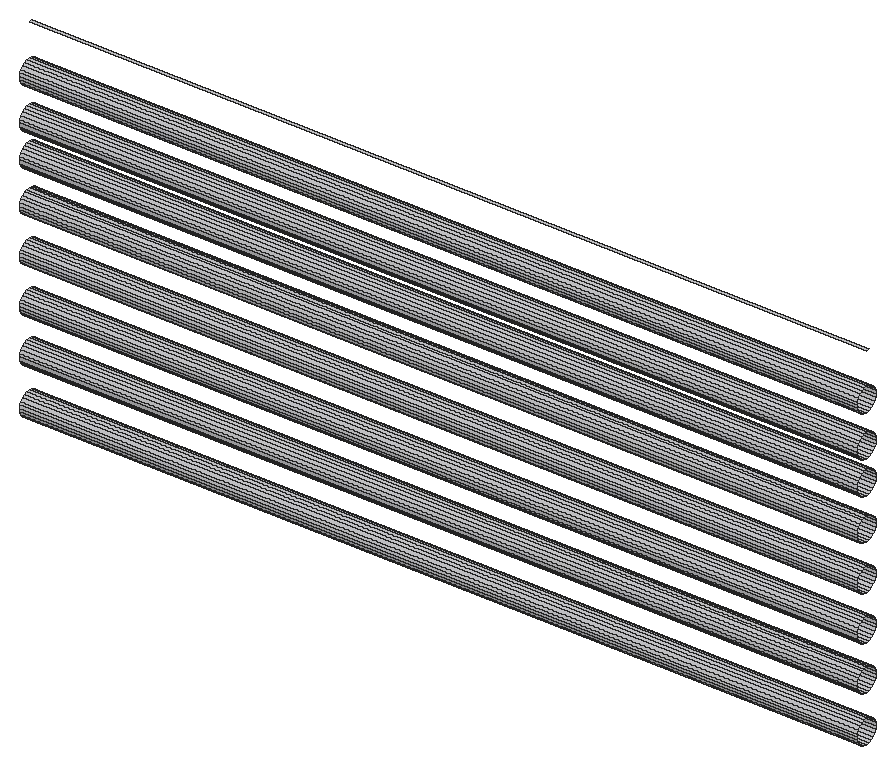
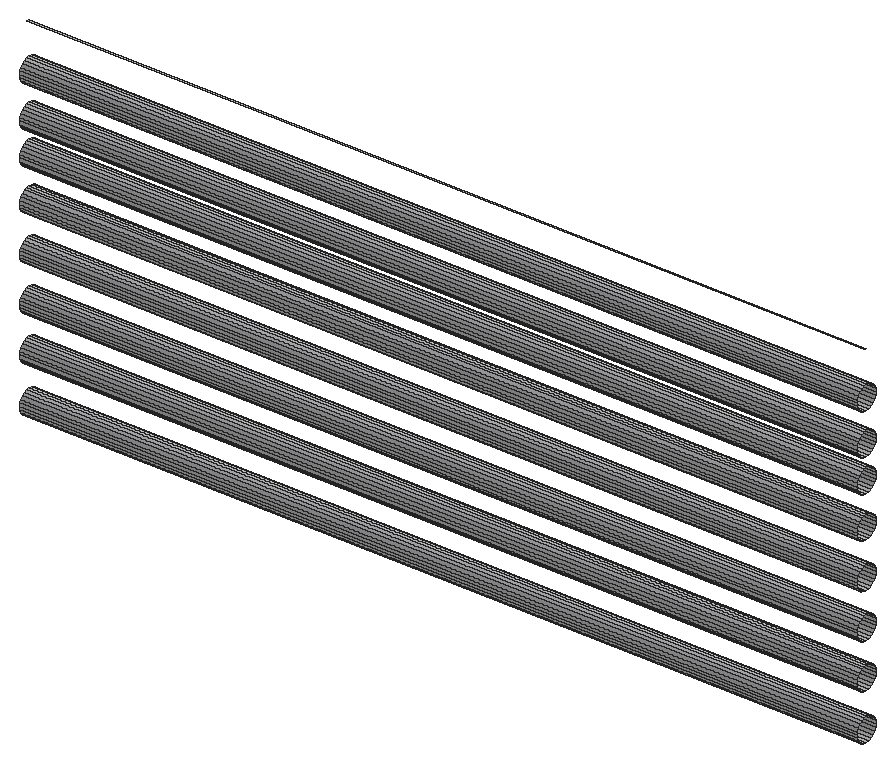
# SketchUp Ruby script. Lengths in inches.
U = 1.inch
M = Sketchup.active_model
def pt(a) = Geom::Point3d.new(a.map { |v| v * U })
def face(e, loops, mat)
  f = e.add_face(loops[0].map { |a| pt(a) })
  loops[1..].each { |l| e.add_face(l.map { |a| pt(a) }).erase! }
  f.material = f.back_material = mat if mat
  f
end
# faces: each face lists its corners as indices into pts; further lists are holes
def faces(e, pts, list, mat = nil) = list.each { |f| face(e, (f[0].is_a?(Array) ? f : [f]).map { |l| l.map { |i| pts[i] } }, mat) }
# xy, xz, yz: faces in a plane at the given z, y or x. An outline is a flat list of corners, or four numbers for a rectangle; further outlines are holes
def ring(l) = l.size == 4 ? [[l[0], l[1]], [l[2], l[1]], [l[2], l[3]], [l[0], l[3]]] : l.each_slice(2).to_a
def flat(e, list, mat, &to3) = list.each { |f| face(e, (f[0].is_a?(Array) ? f : [f]).map { |l| ring(l).map { |u, v| to3.(u, v) } }, mat) }
def xy(e, z, list, mat = nil) = flat(e, list, mat) { |x, y| [x, y, z] }
def xz(e, y, list, mat = nil) = flat(e, list, mat) { |x, z| [x, y, z] }
def yz(e, x, list, mat = nil) = flat(e, list, mat) { |y, z| [x, y, z] }
def lines(e, pts, list) = list.each { |a, b| e.add_line(pt(pts[a]), pt(pts[b])) }
# prism: a flat outline (further loops are holes) pulled along v
def prism(e, loops, v, mat = nil)
  f = face(e, loops, mat); d = Geom::Vector3d.new(v.map { |x| x * U })
  f.pushpull(f.normal.samedirection?(d) ? d.length : -d.length)
end
def box(e, o, s, mat = nil) = prism(e, [[o, [o[0] + s[0], o[1], o[2]], [o[0] + s[0], o[1] + s[1], o[2]], [o[0], o[1] + s[1], o[2]]]], [0, 0, s[2]], mat)
def at(x, y, z, deg = 0) = Geom::Transformation.translation(pt([x, y, z])) * Geom::Transformation.rotation(ORIGIN, Z_AXIS, deg.degrees)
def axes(o, x, y, z) = Geom::Transformation.new([*x, 0, *y, 0, *z, 0, *pt(o).to_a, 1])
def part(name) = M.definitions.add(name)
# library, detail: a bought-in or finely detailed component or shape, given as its bounding box
def library(name, o, s) = part(name).tap { |d| box(d.entities, o, s) }
def detail(e, o, s) = box(e.add_group.entities, o, s)
def put(e, d, t, mat = nil) = e.add_instance(d, t).tap { |i| i.material = mat if mat }
def group(e, t, mat = nil) = e.add_group.tap { |g| g.transformation = t; g.material = mat if mat }.entities
root = M.entities
M.materials.add("[Polished Concrete New]").color = [200, 200, 203]
p = [[204.4,120.13,10.75],[204.4,119.98,10.8125],[160.24,119.98,10.8125],[160.24,120.13,10.75],[204.4,120.29,10.73],[160.24,120.29,10.73],
  [204.4,120.45,10.75],[160.24,120.45,10.75],[204.4,120.6,10.8125],[160.24,120.6,10.8125],[204.4,119.85,10.91],[160.24,119.85,10.91],
  [204.4,120.73,10.91],[160.24,120.73,10.91],[204.4,119.75,11.04],[160.24,119.75,11.04],[204.4,120.83,11.04],[160.24,120.83,11.04],
  [204.4,119.6875,11.19],[160.24,119.6875,11.19],[204.4,120.89,11.19],[160.24,120.89,11.19],[204.4,119.66,11.35],[160.24,119.66,11.35],
  [204.4,120.91,11.35],[160.24,120.91,11.35],[204.4,119.6875,11.51],[160.24,119.6875,11.51],[204.4,120.89,11.51],[160.24,120.89,11.51],
  [204.4,119.75,11.66],[160.24,119.75,11.66],[204.4,120.83,11.66],[160.24,120.83,11.66],[204.4,119.85,11.79],[160.24,119.85,11.79],
  [204.4,120.73,11.79],[160.24,120.73,11.79],[204.4,119.98,11.89],[160.24,119.98,11.89],[204.4,120.6,11.89],[160.24,120.6,11.89],
  [204.4,120.13,11.96],[160.24,120.13,11.96],[204.4,120.45,11.96],[160.24,120.45,11.96],[204.4,120.29,11.98],[160.24,120.29,11.98],
  [204.4,119.98,13.25],[204.4,119.85,13.35],[160.24,119.85,13.35],[160.24,119.98,13.25],[204.4,120.13,13.1875],[160.24,120.13,13.1875],
  [204.4,120.29,13.16],[160.24,120.29,13.16],[204.4,120.45,13.1875],[160.24,120.45,13.1875],[204.4,120.6,13.25],[160.24,120.6,13.25],
  [204.4,120.73,13.35],[160.24,120.73,13.35],[204.4,119.75,13.48],[160.24,119.75,13.48],[204.4,120.83,13.48],[160.24,120.83,13.48],
  [204.4,119.6875,13.63],[160.24,119.6875,13.63],[204.4,120.89,13.63],[160.24,120.89,13.63],[204.4,119.66,13.79],[160.24,119.66,13.79],
  [204.4,120.91,13.79],[160.24,120.91,13.79],[204.4,119.6875,13.95],[160.24,119.6875,13.95],[204.4,120.89,13.95],[160.24,120.89,13.95],
  [204.4,119.75,14.1],[160.24,119.75,14.1],[204.4,120.83,14.1],[160.24,120.83,14.1],[204.4,119.85,14.23],[160.24,119.85,14.23],
  [204.4,120.73,14.23],[160.24,120.73,14.23],[204.4,119.98,14.33],[160.24,119.98,14.33],[204.4,120.6,14.33],[160.24,120.6,14.33],
  [204.4,120.13,14.39],[160.24,120.13,14.39],[204.4,120.45,14.39],[160.24,120.45,14.39],[204.4,120.29,14.41],[160.24,120.29,14.41],
  [204.4,120.29,15.54],[204.4,120.13,15.5625],[160.24,120.13,15.5625],[160.24,120.29,15.54],[204.4,120.45,15.5625],[160.24,120.45,15.5625],
  [204.4,119.98,15.625],[204.4,119.85,15.72],[160.24,119.85,15.72],[160.24,119.98,15.625],[204.4,120.6,15.625],[160.24,120.6,15.625],
  [204.4,120.73,15.72],[160.24,120.73,15.72],[204.4,119.75,15.85],[160.24,119.75,15.85],[204.4,120.83,15.85],[160.24,120.83,15.85],
  [204.4,119.6875,16],[160.24,119.6875,16],[204.4,120.89,16],[160.24,120.89,16],[204.4,119.66,16.16],[160.24,119.66,16.16],
  [204.4,120.91,16.16],[160.24,120.91,16.16],[204.4,119.6875,16.33],[160.24,119.6875,16.33],[204.4,120.89,16.33],[160.24,120.89,16.33],
  [204.4,119.75,16.48],[160.24,119.75,16.48],[204.4,120.83,16.48],[160.24,120.83,16.48],[204.4,119.85,16.61],[160.24,119.85,16.61],
  [204.4,120.73,16.61],[160.24,120.73,16.61],[204.4,119.98,16.71],[160.24,119.98,16.71],[204.4,120.6,16.71],[160.24,120.6,16.71],
  [204.4,120.13,16.77],[160.24,120.13,16.77],[204.4,120.45,16.77],[160.24,120.45,16.77],[204.4,120.29,16.79],[160.24,120.29,16.79],
  [204.4,120.13,17.9375],[204.4,119.98,18],[160.24,119.98,18],[160.24,120.13,17.9375],[204.4,120.29,17.91],[160.24,120.29,17.91],
  [204.4,120.45,17.9375],[160.24,120.45,17.9375],[204.4,120.6,18],[160.24,120.6,18],[204.4,119.85,18.1],[160.24,119.85,18.1],
  [204.4,120.73,18.1],[160.24,120.73,18.1],[204.4,119.75,18.23],[160.24,119.75,18.23],[204.4,120.83,18.23],[160.24,120.83,18.23],
  [204.4,119.6875,18.38],[160.24,119.6875,18.38],[204.4,120.89,18.38],[160.24,120.89,18.38],[204.4,119.66,18.54],[160.24,119.66,18.54],
  [204.4,120.91,18.54],[160.24,120.91,18.54],[204.4,119.6875,18.7],[160.24,119.6875,18.7],[204.4,120.89,18.7],[160.24,120.89,18.7],
  [204.4,119.75,18.85],[160.24,119.75,18.85],[204.4,120.83,18.85],[160.24,120.83,18.85],[204.4,119.85,18.98],[160.24,119.85,18.98],
  [204.4,120.73,18.98],[160.24,120.73,18.98],[204.4,119.98,19.08],[160.24,119.98,19.08],[204.4,120.6,19.08],[160.24,120.6,19.08],
  [204.4,120.13,19.14],[160.24,120.13,19.14],[204.4,120.29,19.16],[160.24,120.29,19.16],[204.4,120.45,19.14],[160.24,120.45,19.14],
  [204.4,120.13,20.3125],[204.4,119.98,20.375],[160.24,119.98,20.375],[160.24,120.13,20.3125],[204.4,120.29,20.29],[160.24,120.29,20.29],
  [204.4,120.45,20.3125],[160.24,120.45,20.3125],[204.4,120.6,20.375],[160.24,120.6,20.375],[204.4,119.85,20.47],[160.24,119.85,20.47],
  [204.4,120.73,20.47],[160.24,120.73,20.47],[204.4,119.75,20.6],[160.24,119.75,20.6],[204.4,120.83,20.6],[160.24,120.83,20.6],
  [204.4,119.6875,20.75],[160.24,119.6875,20.75],[204.4,120.89,20.75],[160.24,120.89,20.75],[204.4,119.66,20.91],[160.24,119.66,20.91],
  [204.4,120.91,20.91],[160.24,120.91,20.91],[204.4,119.6875,21.08],[160.24,119.6875,21.08],[204.4,120.89,21.08],[160.24,120.89,21.08],
  [204.4,119.75,21.23],[160.24,119.75,21.23],[204.4,120.83,21.23],[160.24,120.83,21.23],[204.4,119.85,21.36],[160.24,119.85,21.36],
  [204.4,120.73,21.36],[160.24,120.73,21.36],[204.4,119.98,21.46],[160.24,119.98,21.46],[204.4,120.6,21.46],[160.24,120.6,21.46],
  [204.4,120.13,21.52],[160.24,120.13,21.52],[204.4,120.29,21.54],[160.24,120.29,21.54],[204.4,120.45,21.52],[160.24,120.45,21.52],
  [204.4,120.13,22.5],[204.4,119.98,22.5625],[160.24,119.98,22.5625],[160.24,120.13,22.5],[204.4,120.29,22.48],[160.24,120.29,22.48],
  [204.4,120.45,22.5],[160.24,120.45,22.5],[204.4,120.6,22.5625],[160.24,120.6,22.5625],[204.4,119.85,22.66],[160.24,119.85,22.66],
  [204.4,120.73,22.66],[160.24,120.73,22.66],[204.4,119.75,22.79],[160.24,119.75,22.79],[204.4,120.83,22.79],[160.24,120.83,22.79],
  [204.4,119.6875,22.94],[160.24,119.6875,22.94],[204.4,120.89,22.94],[160.24,120.89,22.94],[204.4,119.66,23.1],[160.24,119.66,23.1],
  [204.4,120.91,23.1],[160.24,120.91,23.1],[204.4,119.6875,23.26],[160.24,119.6875,23.26],[204.4,120.89,23.26],[160.24,120.89,23.26],
  [204.4,119.75,23.41],[160.24,119.75,23.41],[204.4,120.83,23.41],[160.24,120.83,23.41],[204.4,119.85,23.54],[160.24,119.85,23.54],
  [204.4,120.73,23.54],[160.24,120.73,23.54],[204.4,119.98,23.64],[160.24,119.98,23.64],[204.4,120.6,23.64],[160.24,120.6,23.64],
  [204.4,120.13,23.71],[160.24,120.13,23.71],[204.4,120.45,23.71],[160.24,120.45,23.71],[204.4,120.29,23.73],[160.24,120.29,23.73],
  [204.4,120.13,24.25],[204.4,119.98,24.3125],[160.24,119.98,24.3125],[160.24,120.13,24.25],[204.4,120.29,24.23],[160.24,120.29,24.23],
  [204.4,120.45,24.25],[160.24,120.45,24.25],[204.4,120.6,24.3125],[160.24,120.6,24.3125],[204.4,119.85,24.41],[160.24,119.85,24.41],
  [204.4,120.73,24.41],[160.24,120.73,24.41],[204.4,119.75,24.54],[160.24,119.75,24.54],[204.4,120.83,24.54],[160.24,120.83,24.54],
  [204.4,119.6875,24.69],[160.24,119.6875,24.69],[204.4,120.89,24.69],[160.24,120.89,24.69],[204.4,119.66,24.85],[160.24,119.66,24.85],
  [204.4,120.91,24.85],[160.24,120.91,24.85],[204.4,119.6875,25.01],[160.24,119.6875,25.01],[204.4,120.89,25.01],[160.24,120.89,25.01],
  [204.4,119.75,25.16],[160.24,119.75,25.16],[204.4,120.83,25.16],[160.24,120.83,25.16],[204.4,119.85,25.29],[160.24,119.85,25.29],
  [204.4,120.73,25.29],[160.24,120.73,25.29],[204.4,119.98,25.39],[160.24,119.98,25.39],[204.4,120.6,25.39],[160.24,120.6,25.39],
  [204.4,120.13,25.46],[160.24,120.13,25.46],[204.4,120.45,25.46],[160.24,120.45,25.46],[204.4,120.29,25.48],[160.24,120.29,25.48],
  [204.4,120.13,26.4375],[204.4,119.98,26.5],[160.24,119.98,26.5],[160.24,120.13,26.4375],[204.4,120.29,26.41],[160.24,120.29,26.41],
  [204.4,120.45,26.4375],[160.24,120.45,26.4375],[204.4,120.6,26.5],[160.24,120.6,26.5],[204.4,119.85,26.6],[160.24,119.85,26.6],
  [204.4,120.73,26.6],[160.24,120.73,26.6],[204.4,119.75,26.73],[160.24,119.75,26.73],[204.4,120.83,26.73],[160.24,120.83,26.73],
  [204.4,119.6875,26.88],[160.24,119.6875,26.88],[204.4,120.89,26.88],[160.24,120.89,26.88],[204.4,119.66,27.04],[160.24,119.66,27.04],
  [204.4,120.91,27.04],[160.24,120.91,27.04],[204.4,119.6875,27.2],[160.24,119.6875,27.2],[204.4,120.89,27.2],[160.24,120.89,27.2],
  [204.4,119.75,27.35],[160.24,119.75,27.35],[204.4,120.83,27.35],[160.24,120.83,27.35],[204.4,119.85,27.48],[160.24,119.85,27.48],
  [204.4,120.73,27.48],[160.24,120.73,27.48],[204.4,119.98,27.58],[160.24,119.98,27.58],[204.4,120.6,27.58],[160.24,120.6,27.58],
  [204.4,120.13,27.64],[160.24,120.13,27.64],[204.4,120.29,27.66],[160.24,120.29,27.66],[204.4,120.45,27.64],[160.24,120.45,27.64],
  [204.4,120.45,29.375],[204.4,120.29,29.35],[160.24,120.29,29.35],[160.24,120.45,29.375]]
faces(root,p,[[0,1,2,3],[4,0,3,5],[6,4,5,7],[8,6,7,9],[1,10,11,2],[12,8,9,13],[10,14,15,11],[16,12,13,17],
  [14,18,19,15],[20,16,17,21],[18,22,23,19],[24,20,21,25],[22,26,27,23],[28,24,25,29],[26,30,31,27],[32,28,29,33],
  [30,34,35,31],[36,32,33,37],[34,38,39,35],[40,36,37,41],[38,42,43,39],[44,40,41,45],[42,46,47,43],[46,44,45,47],
  [48,49,50,51],[52,48,51,53],[54,52,53,55],[56,54,55,57],[58,56,57,59],[60,58,59,61],[49,62,63,50],[64,60,61,65],
  [62,66,67,63],[68,64,65,69],[66,70,71,67],[72,68,69,73],[70,74,75,71],[76,72,73,77],[74,78,79,75],[80,76,77,81],
  [78,82,83,79],[84,80,81,85],[82,86,87,83],[88,84,85,89],[86,90,91,87],[92,88,89,93],[90,94,95,91],[94,92,93,95],
  [96,97,98,99],[100,96,99,101],[102,103,104,105],[97,102,105,98],[106,100,101,107],[108,106,107,109],[103,110,111,104],[112,108,109,113],
  [110,114,115,111],[116,112,113,117],[114,118,119,115],[120,116,117,121],[118,122,123,119],[124,120,121,125],[122,126,127,123],[128,124,125,129],
  [126,130,131,127],[132,128,129,133],[130,134,135,131],[136,132,133,137],[134,138,139,135],[140,136,137,141],[138,142,143,139],[142,140,141,143],
  [144,145,146,147],[148,144,147,149],[150,148,149,151],[152,150,151,153],[145,154,155,146],[156,152,153,157],[154,158,159,155],[160,156,157,161],
  [158,162,163,159],[164,160,161,165],[162,166,167,163],[168,164,165,169],[166,170,171,167],[172,168,169,173],[170,174,175,171],[176,172,173,177],
  [174,178,179,175],[180,176,177,181],[178,182,183,179],[184,180,181,185],[182,186,187,183],[186,188,189,187],[188,190,191,189],[190,184,185,191],
  [192,193,194,195],[196,192,195,197],[198,196,197,199],[200,198,199,201],[193,202,203,194],[204,200,201,205],[202,206,207,203],[208,204,205,209],
  [206,210,211,207],[212,208,209,213],[210,214,215,211],[216,212,213,217],[214,218,219,215],[220,216,217,221],[218,222,223,219],[224,220,221,225],
  [222,226,227,223],[228,224,225,229],[226,230,231,227],[232,228,229,233],[230,234,235,231],[234,236,237,235],[236,238,239,237],[238,232,233,239],
  [240,241,242,243],[244,240,243,245],[246,244,245,247],[248,246,247,249],[241,250,251,242],[252,248,249,253],[250,254,255,251],[256,252,253,257],
  [254,258,259,255],[260,256,257,261],[258,262,263,259],[264,260,261,265],[262,266,267,263],[268,264,265,269],[266,270,271,267],[272,268,269,273],
  [270,274,275,271],[276,272,273,277],[274,278,279,275],[280,276,277,281],[278,282,283,279],[284,280,281,285],[282,286,287,283],[286,284,285,287],
  [288,289,290,291],[292,288,291,293],[294,292,293,295],[296,294,295,297],[289,298,299,290],[300,296,297,301],[298,302,303,299],[304,300,301,305],
  [302,306,307,303],[308,304,305,309],[306,310,311,307],[312,308,309,313],[310,314,315,311],[316,312,313,317],[314,318,319,315],[320,316,317,321],
  [318,322,323,319],[324,320,321,325],[322,326,327,323],[328,324,325,329],[326,330,331,327],[332,328,329,333],[330,334,335,331],[334,332,333,335],
  [336,337,338,339],[340,336,339,341],[342,340,341,343],[344,342,343,345],[337,346,347,338],[348,344,345,349],[346,350,351,347],[352,348,349,353],
  [350,354,355,351],[356,352,353,357],[354,358,359,355],[360,356,357,361],[358,362,363,359],[364,360,361,365],[362,366,367,363],[368,364,365,369],
  [366,370,371,367],[372,368,369,373],[370,374,375,371],[376,372,373,377],[374,378,379,375],[378,380,381,379],[380,382,383,381],[382,376,377,383],
  [384,385,386,387]],"[Polished Concrete New]")
